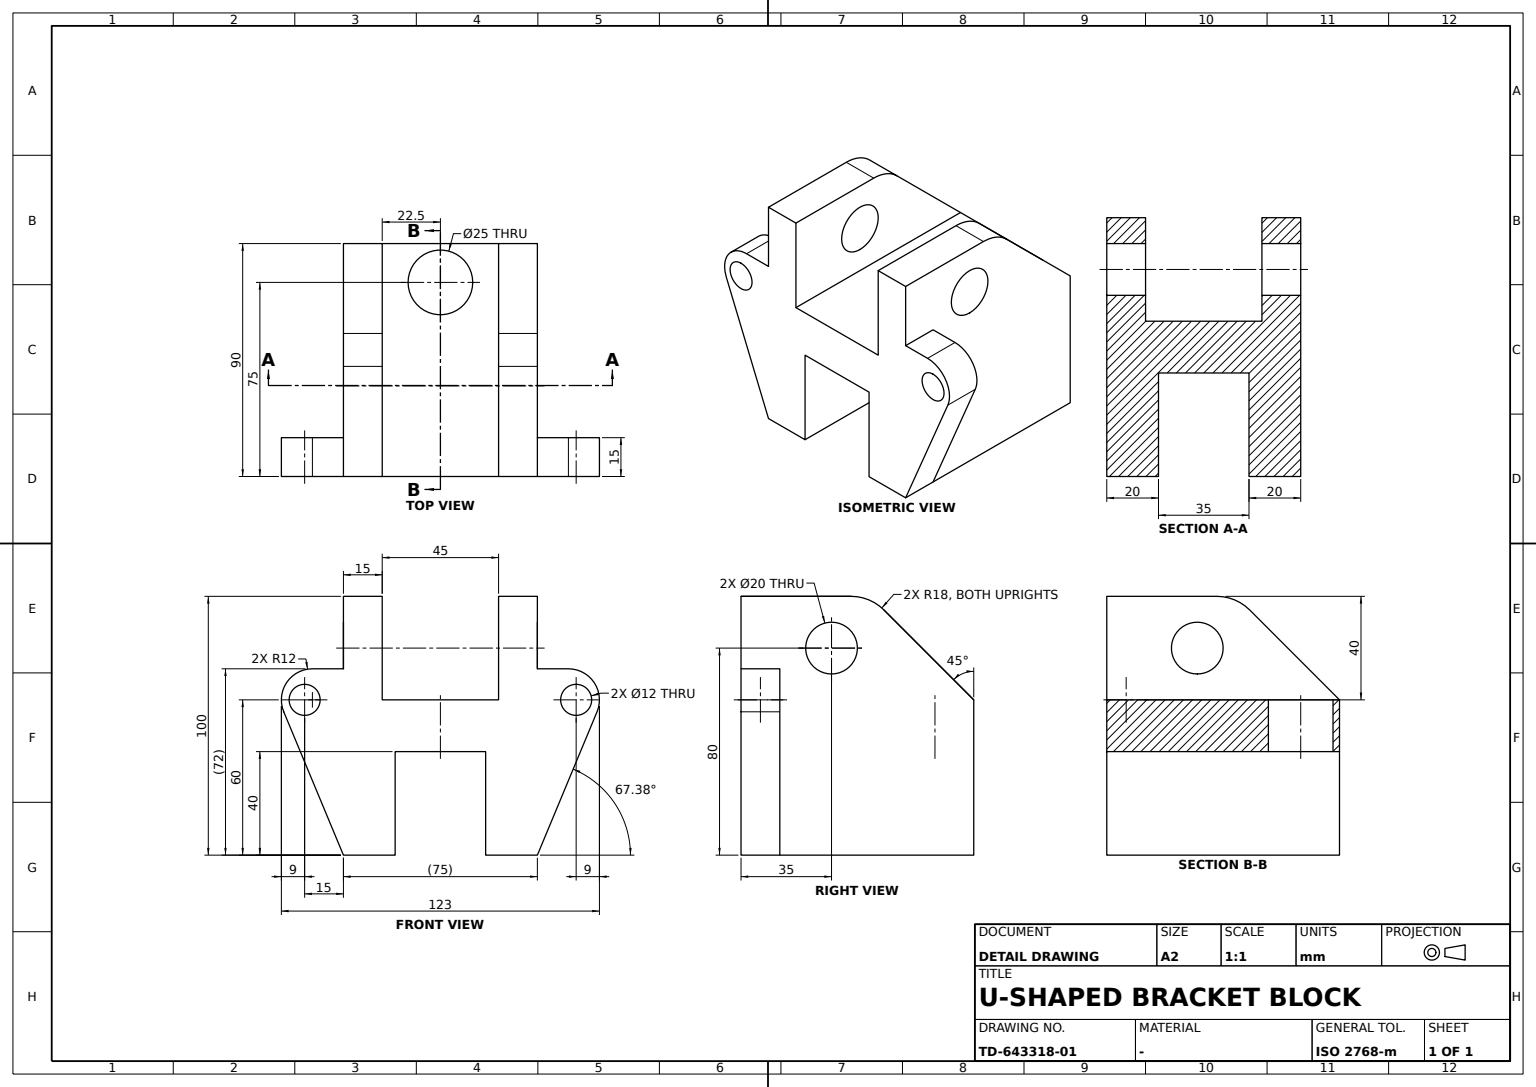
ISO-10303-21;
HEADER;
FILE_DESCRIPTION((''),'2;1');
FILE_NAME('','',(''),(''),'','','');
FILE_SCHEMA(('AUTOMOTIVE_DESIGN'));
ENDSEC;
DATA;
#1=APPLICATION_CONTEXT('');
#2=PRODUCT_CONTEXT('',#1,'mechanical');
#3=PRODUCT('','','',(#2));
#4=PRODUCT_DEFINITION_FORMATION('','',#3);
#5=PRODUCT_DEFINITION_CONTEXT('',#1,'design');
#6=PRODUCT_DEFINITION('','',#4,#5);
#7=PRODUCT_DEFINITION_SHAPE('','',#6);
#8=(LENGTH_UNIT()NAMED_UNIT(*)SI_UNIT(.MILLI.,.METRE.));
#9=(NAMED_UNIT(*)PLANE_ANGLE_UNIT()SI_UNIT($,.RADIAN.));
#10=(NAMED_UNIT(*)SI_UNIT($,.STERADIAN.)SOLID_ANGLE_UNIT());
#11=UNCERTAINTY_MEASURE_WITH_UNIT(LENGTH_MEASURE(0.005),#8,'distance_accuracy_value','');
#12=(GEOMETRIC_REPRESENTATION_CONTEXT(3)GLOBAL_UNCERTAINTY_ASSIGNED_CONTEXT((#11))GLOBAL_UNIT_ASSIGNED_CONTEXT((#8,#9,#10))REPRESENTATION_CONTEXT('',''));
#13=CARTESIAN_POINT('',(60.576923,-45.,15.384615));
#14=VERTEX_POINT('',#13);
#15=CARTESIAN_POINT('',(60.576923,-30.,15.384615));
#16=VERTEX_POINT('',#15);
#17=CARTESIAN_POINT('',(60.576923,-37.5,15.384615));
#18=DIRECTION('',(0.,1.,0.));
#19=VECTOR('',#18,1000.);
#20=LINE('',#17,#19);
#21=EDGE_CURVE('',#14,#16,#20,.T.);
#22=ORIENTED_EDGE('',*,*,#21,.F.);
#23=CARTESIAN_POINT('',(37.5,-45.,-40.));
#24=VERTEX_POINT('',#23);
#25=CARTESIAN_POINT('',(46.153846,-45.,-19.230769));
#26=DIRECTION('',(-0.384615385,0.,-0.923076923));
#27=VECTOR('',#26,1000.);
#28=LINE('',#25,#27);
#29=EDGE_CURVE('',#14,#24,#28,.T.);
#30=ORIENTED_EDGE('',*,*,#29,.T.);
#31=CARTESIAN_POINT('',(37.5,-30.,-40.));
#32=VERTEX_POINT('',#31);
#33=CARTESIAN_POINT('',(37.5,0.,-40.));
#34=LINE('',#33,#19);
#35=EDGE_CURVE('',#24,#32,#34,.T.);
#36=ORIENTED_EDGE('',*,*,#35,.T.);
#37=CARTESIAN_POINT('',(67.5,-30.,32.));
#38=LINE('',#37,#27);
#39=EDGE_CURVE('',#16,#32,#38,.T.);
#40=ORIENTED_EDGE('',*,*,#39,.F.);
#41=EDGE_LOOP('',(#22,#30,#36,#40));
#42=FACE_BOUND('',#41,.T.);
#43=CARTESIAN_POINT('',(67.5,-45.,32.));
#44=DIRECTION('',(0.923076923,0.,-0.384615385));
#45=AXIS2_PLACEMENT_3D('',#43,#44,#26);
#46=PLANE('',#45);
#47=ADVANCED_FACE('',(#42),#46,.T.);
#48=CARTESIAN_POINT('',(-22.5,-10.,30.));
#49=VERTEX_POINT('',#48);
#50=CARTESIAN_POINT('',(-22.5,-10.,40.));
#51=DIRECTION('',(1.,0.,0.));
#52=DIRECTION('',(0.,0.,-1.));
#53=AXIS2_PLACEMENT_3D('',#50,#51,#52);
#54=CIRCLE('',#53,10.);
#55=EDGE_CURVE('',#49,#49,#54,.T.);
#56=ORIENTED_EDGE('',*,*,#55,.T.);
#57=EDGE_LOOP('',(#56));
#58=FACE_BOUND('',#57,.T.);
#59=CARTESIAN_POINT('',(-37.5,-10.,30.));
#60=VERTEX_POINT('',#59);
#61=CARTESIAN_POINT('',(-37.5,-10.,40.));
#62=AXIS2_PLACEMENT_3D('',#61,#51,#52);
#63=CIRCLE('',#62,10.);
#64=EDGE_CURVE('',#60,#60,#63,.T.);
#65=ORIENTED_EDGE('',*,*,#64,.F.);
#66=EDGE_LOOP('',(#65));
#67=FACE_BOUND('',#66,.T.);
#68=CARTESIAN_POINT('',(30.,-10.,40.));
#69=AXIS2_PLACEMENT_3D('',#68,#51,#18);
#70=CYLINDRICAL_SURFACE('',#69,10.);
#71=ADVANCED_FACE('',(#58,#67),#70,.F.);
#72=CARTESIAN_POINT('',(-12.5,30.,20.));
#73=VERTEX_POINT('',#72);
#74=CARTESIAN_POINT('',(0.,30.,20.));
#75=DIRECTION('',(-1.,0.,0.));
#76=AXIS2_PLACEMENT_3D('',#74,#52,#75);
#77=CIRCLE('',#76,12.5);
#78=EDGE_CURVE('',#73,#73,#77,.F.);
#79=ORIENTED_EDGE('',*,*,#78,.T.);
#80=EDGE_LOOP('',(#79));
#81=FACE_BOUND('',#80,.T.);
#82=CARTESIAN_POINT('',(12.5,30.,0.));
#83=VERTEX_POINT('',#82);
#84=CARTESIAN_POINT('',(0.,30.,0.));
#85=DIRECTION('',(0.,0.,1.));
#86=AXIS2_PLACEMENT_3D('',#84,#85,#51);
#87=CIRCLE('',#86,12.5);
#88=EDGE_CURVE('',#83,#83,#87,.T.);
#89=ORIENTED_EDGE('',*,*,#88,.F.);
#90=EDGE_LOOP('',(#89));
#91=FACE_BOUND('',#90,.T.);
#92=CARTESIAN_POINT('',(0.,30.,10.));
#93=AXIS2_PLACEMENT_3D('',#92,#85,#18);
#94=CYLINDRICAL_SURFACE('',#93,12.5);
#95=ADVANCED_FACE('',(#81,#91),#94,.F.);
#96=CARTESIAN_POINT('',(37.5,-10.,50.));
#97=VERTEX_POINT('',#96);
#98=CARTESIAN_POINT('',(37.5,-10.,40.));
#99=AXIS2_PLACEMENT_3D('',#98,#75,#85);
#100=CIRCLE('',#99,10.);
#101=EDGE_CURVE('',#97,#97,#100,.F.);
#102=ORIENTED_EDGE('',*,*,#101,.T.);
#103=EDGE_LOOP('',(#102));
#104=FACE_BOUND('',#103,.T.);
#105=CARTESIAN_POINT('',(22.5,-10.,30.));
#106=VERTEX_POINT('',#105);
#107=CARTESIAN_POINT('',(22.5,-10.,40.));
#108=AXIS2_PLACEMENT_3D('',#107,#51,#52);
#109=CIRCLE('',#108,10.);
#110=EDGE_CURVE('',#106,#106,#109,.T.);
#111=ORIENTED_EDGE('',*,*,#110,.F.);
#112=EDGE_LOOP('',(#111));
#113=FACE_BOUND('',#112,.T.);
#114=ADVANCED_FACE('',(#104,#113),#70,.F.);
#115=CARTESIAN_POINT('',(-22.5,10.272078,54.727922));
#116=VERTEX_POINT('',#115);
#117=CARTESIAN_POINT('',(-37.5,10.272078,54.727922));
#118=VERTEX_POINT('',#117);
#119=CARTESIAN_POINT('',(-30.,10.272078,54.727922));
#120=VECTOR('',#75,1000.);
#121=LINE('',#119,#120);
#122=EDGE_CURVE('',#116,#118,#121,.T.);
#123=ORIENTED_EDGE('',*,*,#122,.T.);
#124=CARTESIAN_POINT('',(-37.5,-2.455844,60.));
#125=VERTEX_POINT('',#124);
#126=CARTESIAN_POINT('',(-37.5,-2.455844,42.));
#127=AXIS2_PLACEMENT_3D('',#126,#51,#52);
#128=CIRCLE('',#127,18.);
#129=EDGE_CURVE('',#118,#125,#128,.T.);
#130=ORIENTED_EDGE('',*,*,#129,.T.);
#131=CARTESIAN_POINT('',(-22.5,-2.455844,60.));
#132=VERTEX_POINT('',#131);
#133=CARTESIAN_POINT('',(-30.,-2.455844,60.));
#134=LINE('',#133,#120);
#135=EDGE_CURVE('',#132,#125,#134,.T.);
#136=ORIENTED_EDGE('',*,*,#135,.F.);
#137=CARTESIAN_POINT('',(-22.5,-2.455844,42.));
#138=AXIS2_PLACEMENT_3D('',#137,#51,#52);
#139=CIRCLE('',#138,18.);
#140=EDGE_CURVE('',#116,#132,#139,.T.);
#141=ORIENTED_EDGE('',*,*,#140,.F.);
#142=EDGE_LOOP('',(#123,#130,#136,#141));
#143=FACE_BOUND('',#142,.T.);
#144=CARTESIAN_POINT('',(-30.,-2.455844,42.));
#145=AXIS2_PLACEMENT_3D('',#144,#75,#85);
#146=CYLINDRICAL_SURFACE('',#145,18.);
#147=ADVANCED_FACE('',(#143),#146,.T.);
#148=ORIENTED_EDGE('',*,*,#122,.F.);
#149=CARTESIAN_POINT('',(-22.5,45.,20.));
#150=VERTEX_POINT('',#149);
#151=CARTESIAN_POINT('',(-22.5,5.,60.));
#152=DIRECTION('',(0.,0.707106781,-0.707106781));
#153=VECTOR('',#152,1000.);
#154=LINE('',#151,#153);
#155=EDGE_CURVE('',#116,#150,#154,.T.);
#156=ORIENTED_EDGE('',*,*,#155,.T.);
#157=CARTESIAN_POINT('',(-37.5,45.,20.));
#158=VERTEX_POINT('',#157);
#159=CARTESIAN_POINT('',(0.,45.,20.));
#160=VECTOR('',#51,1000.);
#161=LINE('',#159,#160);
#162=EDGE_CURVE('',#158,#150,#161,.T.);
#163=ORIENTED_EDGE('',*,*,#162,.F.);
#164=CARTESIAN_POINT('',(-37.5,5.,60.));
#165=LINE('',#164,#153);
#166=EDGE_CURVE('',#118,#158,#165,.T.);
#167=ORIENTED_EDGE('',*,*,#166,.F.);
#168=EDGE_LOOP('',(#148,#156,#163,#167));
#169=FACE_BOUND('',#168,.T.);
#170=CARTESIAN_POINT('',(37.5,5.,60.));
#171=DIRECTION('',(0.,0.707106781,0.707106781));
#172=AXIS2_PLACEMENT_3D('',#170,#171,#152);
#173=PLANE('',#172);
#174=ADVANCED_FACE('',(#169),#173,.T.);
#175=CARTESIAN_POINT('',(17.5,45.,0.));
#176=VERTEX_POINT('',#175);
#177=CARTESIAN_POINT('',(17.5,45.,-40.));
#178=VERTEX_POINT('',#177);
#179=VECTOR('',#52,1000.);
#180=LINE('',#175,#179);
#181=EDGE_CURVE('',#176,#178,#180,.T.);
#182=ORIENTED_EDGE('',*,*,#181,.F.);
#183=CARTESIAN_POINT('',(-17.5,45.,0.));
#184=VERTEX_POINT('',#183);
#185=CARTESIAN_POINT('',(0.,45.,0.));
#186=LINE('',#185,#160);
#187=EDGE_CURVE('',#184,#176,#186,.T.);
#188=ORIENTED_EDGE('',*,*,#187,.F.);
#189=CARTESIAN_POINT('',(-17.5,45.,-40.));
#190=VERTEX_POINT('',#189);
#191=VECTOR('',#85,1000.);
#192=LINE('',#183,#191);
#193=EDGE_CURVE('',#190,#184,#192,.T.);
#194=ORIENTED_EDGE('',*,*,#193,.F.);
#195=CARTESIAN_POINT('',(-37.5,45.,-40.));
#196=VERTEX_POINT('',#195);
#197=CARTESIAN_POINT('',(0.,45.,-40.));
#198=LINE('',#197,#160);
#199=EDGE_CURVE('',#196,#190,#198,.T.);
#200=ORIENTED_EDGE('',*,*,#199,.F.);
#201=CARTESIAN_POINT('',(-37.5,45.,0.));
#202=LINE('',#201,#179);
#203=EDGE_CURVE('',#158,#196,#202,.T.);
#204=ORIENTED_EDGE('',*,*,#203,.F.);
#205=ORIENTED_EDGE('',*,*,#162,.T.);
#206=CARTESIAN_POINT('',(22.5,45.,20.));
#207=VERTEX_POINT('',#206);
#208=LINE('',#159,#120);
#209=EDGE_CURVE('',#207,#150,#208,.T.);
#210=ORIENTED_EDGE('',*,*,#209,.F.);
#211=CARTESIAN_POINT('',(37.5,45.,20.));
#212=VERTEX_POINT('',#211);
#213=LINE('',#211,#120);
#214=EDGE_CURVE('',#212,#207,#213,.T.);
#215=ORIENTED_EDGE('',*,*,#214,.F.);
#216=CARTESIAN_POINT('',(37.5,45.,-40.));
#217=VERTEX_POINT('',#216);
#218=CARTESIAN_POINT('',(37.5,45.,0.));
#219=LINE('',#218,#191);
#220=EDGE_CURVE('',#217,#212,#219,.T.);
#221=ORIENTED_EDGE('',*,*,#220,.F.);
#222=EDGE_CURVE('',#178,#217,#198,.T.);
#223=ORIENTED_EDGE('',*,*,#222,.F.);
#224=EDGE_LOOP('',(#182,#188,#194,#200,#204,#205,#210,#215,#221,#223));
#225=FACE_BOUND('',#224,.T.);
#226=AXIS2_PLACEMENT_3D('',#185,#18,#75);
#227=PLANE('',#226);
#228=ADVANCED_FACE('',(#225),#227,.T.);
#229=CARTESIAN_POINT('',(-37.5,-45.,-40.));
#230=VERTEX_POINT('',#229);
#231=CARTESIAN_POINT('',(-17.5,-45.,-40.));
#232=VERTEX_POINT('',#231);
#233=CARTESIAN_POINT('',(0.,-45.,-40.));
#234=LINE('',#233,#160);
#235=EDGE_CURVE('',#230,#232,#234,.T.);
#236=ORIENTED_EDGE('',*,*,#235,.F.);
#237=CARTESIAN_POINT('',(-37.5,-30.,-40.));
#238=VERTEX_POINT('',#237);
#239=CARTESIAN_POINT('',(-37.5,0.,-40.));
#240=LINE('',#239,#19);
#241=EDGE_CURVE('',#230,#238,#240,.T.);
#242=ORIENTED_EDGE('',*,*,#241,.T.);
#243=EDGE_CURVE('',#238,#196,#240,.T.);
#244=ORIENTED_EDGE('',*,*,#243,.T.);
#245=ORIENTED_EDGE('',*,*,#199,.T.);
#246=CARTESIAN_POINT('',(-17.5,0.,-40.));
#247=LINE('',#246,#19);
#248=EDGE_CURVE('',#232,#190,#247,.T.);
#249=ORIENTED_EDGE('',*,*,#248,.F.);
#250=EDGE_LOOP('',(#236,#242,#244,#245,#249));
#251=FACE_BOUND('',#250,.T.);
#252=AXIS2_PLACEMENT_3D('',#239,#85,#51);
#253=PLANE('',#252);
#254=ADVANCED_FACE('',(#251),#253,.F.);
#255=CARTESIAN_POINT('',(-37.5,-45.,60.));
#256=VERTEX_POINT('',#255);
#257=CARTESIAN_POINT('',(-22.5,-45.,60.));
#258=VERTEX_POINT('',#257);
#259=CARTESIAN_POINT('',(0.,-45.,60.));
#260=LINE('',#259,#160);
#261=EDGE_CURVE('',#256,#258,#260,.T.);
#262=ORIENTED_EDGE('',*,*,#261,.T.);
#263=LINE('',#257,#19);
#264=EDGE_CURVE('',#258,#132,#263,.T.);
#265=ORIENTED_EDGE('',*,*,#264,.T.);
#266=ORIENTED_EDGE('',*,*,#135,.T.);
#267=LINE('',#255,#19);
#268=EDGE_CURVE('',#256,#125,#267,.T.);
#269=ORIENTED_EDGE('',*,*,#268,.F.);
#270=EDGE_LOOP('',(#262,#265,#266,#269));
#271=FACE_BOUND('',#270,.T.);
#272=CARTESIAN_POINT('',(37.5,-45.,60.));
#273=AXIS2_PLACEMENT_3D('',#272,#85,#18);
#274=PLANE('',#273);
#275=ADVANCED_FACE('',(#271),#274,.T.);
#276=ORIENTED_EDGE('',*,*,#264,.F.);
#277=CARTESIAN_POINT('',(-22.5,-45.,20.));
#278=VERTEX_POINT('',#277);
#279=CARTESIAN_POINT('',(-22.5,-45.,0.));
#280=LINE('',#279,#191);
#281=EDGE_CURVE('',#278,#258,#280,.T.);
#282=ORIENTED_EDGE('',*,*,#281,.F.);
#283=CARTESIAN_POINT('',(-22.5,0.,20.));
#284=DIRECTION('',(0.,-1.,0.));
#285=VECTOR('',#284,1000.);
#286=LINE('',#283,#285);
#287=EDGE_CURVE('',#150,#278,#286,.T.);
#288=ORIENTED_EDGE('',*,*,#287,.F.);
#289=ORIENTED_EDGE('',*,*,#155,.F.);
#290=ORIENTED_EDGE('',*,*,#140,.T.);
#291=EDGE_LOOP('',(#276,#282,#288,#289,#290));
#292=FACE_BOUND('',#291,.T.);
#293=ORIENTED_EDGE('',*,*,#55,.F.);
#294=EDGE_LOOP('',(#293));
#295=FACE_BOUND('',#294,.T.);
#296=CARTESIAN_POINT('',(-22.5,0.,0.));
#297=AXIS2_PLACEMENT_3D('',#296,#51,#18);
#298=PLANE('',#297);
#299=ADVANCED_FACE('',(#292,#295),#298,.T.);
#300=VERTEX_POINT('',#272);
#301=CARTESIAN_POINT('',(37.5,-2.455844,60.));
#302=VERTEX_POINT('',#301);
#303=CARTESIAN_POINT('',(37.5,0.,60.));
#304=LINE('',#303,#19);
#305=EDGE_CURVE('',#300,#302,#304,.T.);
#306=ORIENTED_EDGE('',*,*,#305,.F.);
#307=CARTESIAN_POINT('',(37.5,-45.,32.));
#308=VERTEX_POINT('',#307);
#309=CARTESIAN_POINT('',(37.5,-45.,0.));
#310=LINE('',#309,#191);
#311=EDGE_CURVE('',#308,#300,#310,.T.);
#312=ORIENTED_EDGE('',*,*,#311,.F.);
#313=CARTESIAN_POINT('',(37.5,-30.,32.));
#314=VERTEX_POINT('',#313);
#315=CARTESIAN_POINT('',(37.5,0.,32.));
#316=LINE('',#315,#19);
#317=EDGE_CURVE('',#308,#314,#316,.T.);
#318=ORIENTED_EDGE('',*,*,#317,.T.);
#319=LINE('',#31,#191);
#320=EDGE_CURVE('',#32,#314,#319,.T.);
#321=ORIENTED_EDGE('',*,*,#320,.F.);
#322=EDGE_CURVE('',#32,#217,#34,.T.);
#323=ORIENTED_EDGE('',*,*,#322,.T.);
#324=ORIENTED_EDGE('',*,*,#220,.T.);
#325=CARTESIAN_POINT('',(37.5,10.272078,54.727922));
#326=VERTEX_POINT('',#325);
#327=CARTESIAN_POINT('',(37.5,52.5,12.5));
#328=LINE('',#327,#153);
#329=EDGE_CURVE('',#326,#212,#328,.T.);
#330=ORIENTED_EDGE('',*,*,#329,.F.);
#331=CARTESIAN_POINT('',(37.5,-2.455844,42.));
#332=AXIS2_PLACEMENT_3D('',#331,#75,#85);
#333=CIRCLE('',#332,18.);
#334=EDGE_CURVE('',#302,#326,#333,.T.);
#335=ORIENTED_EDGE('',*,*,#334,.F.);
#336=EDGE_LOOP('',(#306,#312,#318,#321,#323,#324,#330,#335));
#337=FACE_BOUND('',#336,.T.);
#338=ORIENTED_EDGE('',*,*,#101,.F.);
#339=EDGE_LOOP('',(#338));
#340=FACE_BOUND('',#339,.T.);
#341=AXIS2_PLACEMENT_3D('',#33,#75,#85);
#342=PLANE('',#341);
#343=ADVANCED_FACE('',(#337,#340),#342,.F.);
#344=CARTESIAN_POINT('',(-37.5,-45.,32.));
#345=VERTEX_POINT('',#344);
#346=CARTESIAN_POINT('',(-37.5,-30.,32.));
#347=VERTEX_POINT('',#346);
#348=LINE('',#344,#19);
#349=EDGE_CURVE('',#345,#347,#348,.T.);
#350=ORIENTED_EDGE('',*,*,#349,.F.);
#351=CARTESIAN_POINT('',(-37.5,-45.,0.));
#352=LINE('',#351,#179);
#353=EDGE_CURVE('',#256,#345,#352,.T.);
#354=ORIENTED_EDGE('',*,*,#353,.F.);
#355=ORIENTED_EDGE('',*,*,#268,.T.);
#356=ORIENTED_EDGE('',*,*,#129,.F.);
#357=ORIENTED_EDGE('',*,*,#166,.T.);
#358=ORIENTED_EDGE('',*,*,#203,.T.);
#359=ORIENTED_EDGE('',*,*,#243,.F.);
#360=CARTESIAN_POINT('',(-37.5,-30.,0.));
#361=LINE('',#360,#191);
#362=EDGE_CURVE('',#238,#347,#361,.T.);
#363=ORIENTED_EDGE('',*,*,#362,.T.);
#364=EDGE_LOOP('',(#350,#354,#355,#356,#357,#358,#359,#363));
#365=FACE_BOUND('',#364,.T.);
#366=ORIENTED_EDGE('',*,*,#64,.T.);
#367=EDGE_LOOP('',(#366));
#368=FACE_BOUND('',#367,.T.);
#369=CARTESIAN_POINT('',(-37.5,0.,20.));
#370=AXIS2_PLACEMENT_3D('',#369,#51,#52);
#371=PLANE('',#370);
#372=ADVANCED_FACE('',(#365,#368),#371,.F.);
#373=CARTESIAN_POINT('',(22.5,10.272078,54.727922));
#374=VERTEX_POINT('',#373);
#375=CARTESIAN_POINT('',(22.5,5.,60.));
#376=LINE('',#375,#153);
#377=EDGE_CURVE('',#374,#207,#376,.T.);
#378=ORIENTED_EDGE('',*,*,#377,.F.);
#379=EDGE_CURVE('',#326,#374,#121,.T.);
#380=ORIENTED_EDGE('',*,*,#379,.F.);
#381=ORIENTED_EDGE('',*,*,#329,.T.);
#382=ORIENTED_EDGE('',*,*,#214,.T.);
#383=EDGE_LOOP('',(#378,#380,#381,#382));
#384=FACE_BOUND('',#383,.T.);
#385=ADVANCED_FACE('',(#384),#173,.T.);
#386=CARTESIAN_POINT('',(17.5,-45.,0.));
#387=VERTEX_POINT('',#386);
#388=CARTESIAN_POINT('',(17.5,-45.,-40.));
#389=VERTEX_POINT('',#388);
#390=LINE('',#386,#179);
#391=EDGE_CURVE('',#387,#389,#390,.T.);
#392=ORIENTED_EDGE('',*,*,#391,.F.);
#393=CARTESIAN_POINT('',(17.5,0.,0.));
#394=LINE('',#393,#19);
#395=EDGE_CURVE('',#387,#176,#394,.T.);
#396=ORIENTED_EDGE('',*,*,#395,.T.);
#397=ORIENTED_EDGE('',*,*,#181,.T.);
#398=CARTESIAN_POINT('',(17.5,0.,-40.));
#399=LINE('',#398,#19);
#400=EDGE_CURVE('',#389,#178,#399,.T.);
#401=ORIENTED_EDGE('',*,*,#400,.F.);
#402=EDGE_LOOP('',(#392,#396,#397,#401));
#403=FACE_BOUND('',#402,.T.);
#404=AXIS2_PLACEMENT_3D('',#393,#51,#52);
#405=PLANE('',#404);
#406=ADVANCED_FACE('',(#403),#405,.F.);
#407=ORIENTED_EDGE('',*,*,#349,.T.);
#408=CARTESIAN_POINT('',(-49.5,-30.,32.));
#409=VERTEX_POINT('',#408);
#410=CARTESIAN_POINT('',(0.,-30.,32.));
#411=LINE('',#410,#120);
#412=EDGE_CURVE('',#347,#409,#411,.T.);
#413=ORIENTED_EDGE('',*,*,#412,.T.);
#414=CARTESIAN_POINT('',(-49.5,-45.,32.));
#415=VERTEX_POINT('',#414);
#416=CARTESIAN_POINT('',(-49.5,-37.5,32.));
#417=LINE('',#416,#19);
#418=EDGE_CURVE('',#415,#409,#417,.T.);
#419=ORIENTED_EDGE('',*,*,#418,.F.);
#420=LINE('',#307,#120);
#421=EDGE_CURVE('',#345,#415,#420,.T.);
#422=ORIENTED_EDGE('',*,*,#421,.F.);
#423=EDGE_LOOP('',(#407,#413,#419,#422));
#424=FACE_BOUND('',#423,.T.);
#425=AXIS2_PLACEMENT_3D('',#307,#85,#51);
#426=PLANE('',#425);
#427=ADVANCED_FACE('',(#424),#426,.T.);
#428=ORIENTED_EDGE('',*,*,#261,.F.);
#429=ORIENTED_EDGE('',*,*,#353,.T.);
#430=ORIENTED_EDGE('',*,*,#421,.T.);
#431=CARTESIAN_POINT('',(-60.576923,-45.,15.384615));
#432=VERTEX_POINT('',#431);
#433=CARTESIAN_POINT('',(-49.5,-45.,20.));
#434=AXIS2_PLACEMENT_3D('',#433,#18,#85);
#435=CIRCLE('',#434,12.);
#436=EDGE_CURVE('',#432,#415,#435,.T.);
#437=ORIENTED_EDGE('',*,*,#436,.F.);
#438=CARTESIAN_POINT('',(-46.153846,-45.,-19.230769));
#439=DIRECTION('',(0.384615385,0.,-0.923076923));
#440=VECTOR('',#439,1000.);
#441=LINE('',#438,#440);
#442=EDGE_CURVE('',#432,#230,#441,.T.);
#443=ORIENTED_EDGE('',*,*,#442,.T.);
#444=ORIENTED_EDGE('',*,*,#235,.T.);
#445=CARTESIAN_POINT('',(-17.5,-45.,0.));
#446=VERTEX_POINT('',#445);
#447=LINE('',#445,#191);
#448=EDGE_CURVE('',#232,#446,#447,.T.);
#449=ORIENTED_EDGE('',*,*,#448,.T.);
#450=CARTESIAN_POINT('',(0.,-45.,0.));
#451=LINE('',#450,#160);
#452=EDGE_CURVE('',#446,#387,#451,.T.);
#453=ORIENTED_EDGE('',*,*,#452,.T.);
#454=ORIENTED_EDGE('',*,*,#391,.T.);
#455=EDGE_CURVE('',#389,#24,#234,.T.);
#456=ORIENTED_EDGE('',*,*,#455,.T.);
#457=ORIENTED_EDGE('',*,*,#29,.F.);
#458=CARTESIAN_POINT('',(49.5,-45.,32.));
#459=VERTEX_POINT('',#458);
#460=CARTESIAN_POINT('',(49.5,-45.,20.));
#461=AXIS2_PLACEMENT_3D('',#460,#18,#85);
#462=CIRCLE('',#461,12.);
#463=EDGE_CURVE('',#459,#14,#462,.T.);
#464=ORIENTED_EDGE('',*,*,#463,.F.);
#465=CARTESIAN_POINT('',(0.,-45.,32.));
#466=LINE('',#465,#160);
#467=EDGE_CURVE('',#308,#459,#466,.T.);
#468=ORIENTED_EDGE('',*,*,#467,.F.);
#469=ORIENTED_EDGE('',*,*,#311,.T.);
#470=CARTESIAN_POINT('',(22.5,-45.,60.));
#471=VERTEX_POINT('',#470);
#472=LINE('',#272,#120);
#473=EDGE_CURVE('',#300,#471,#472,.T.);
#474=ORIENTED_EDGE('',*,*,#473,.T.);
#475=CARTESIAN_POINT('',(22.5,-45.,20.));
#476=VERTEX_POINT('',#475);
#477=CARTESIAN_POINT('',(22.5,-45.,0.));
#478=LINE('',#477,#191);
#479=EDGE_CURVE('',#476,#471,#478,.T.);
#480=ORIENTED_EDGE('',*,*,#479,.F.);
#481=CARTESIAN_POINT('',(0.,-45.,20.));
#482=LINE('',#481,#120);
#483=EDGE_CURVE('',#476,#278,#482,.T.);
#484=ORIENTED_EDGE('',*,*,#483,.T.);
#485=ORIENTED_EDGE('',*,*,#281,.T.);
#486=EDGE_LOOP('',(#428,#429,#430,#437,#443,#444,#449,#453,#454,#456,#457,#464,#468,#469,#474,#480,#484,#485));
#487=FACE_BOUND('',#486,.T.);
#488=CARTESIAN_POINT('',(-52.5,-45.,26.));
#489=VERTEX_POINT('',#488);
#490=CARTESIAN_POINT('',(-52.5,-45.,20.));
#491=AXIS2_PLACEMENT_3D('',#490,#18,#85);
#492=CIRCLE('',#491,6.);
#493=EDGE_CURVE('',#489,#489,#492,.T.);
#494=ORIENTED_EDGE('',*,*,#493,.T.);
#495=EDGE_LOOP('',(#494));
#496=FACE_BOUND('',#495,.T.);
#497=CARTESIAN_POINT('',(52.5,-45.,26.));
#498=VERTEX_POINT('',#497);
#499=CARTESIAN_POINT('',(52.5,-45.,20.));
#500=AXIS2_PLACEMENT_3D('',#499,#18,#85);
#501=CIRCLE('',#500,6.);
#502=EDGE_CURVE('',#498,#498,#501,.F.);
#503=ORIENTED_EDGE('',*,*,#502,.F.);
#504=EDGE_LOOP('',(#503));
#505=FACE_BOUND('',#504,.T.);
#506=AXIS2_PLACEMENT_3D('',#450,#18,#75);
#507=PLANE('',#506);
#508=ADVANCED_FACE('',(#487,#496,#505),#507,.F.);
#509=ORIENTED_EDGE('',*,*,#110,.T.);
#510=EDGE_LOOP('',(#509));
#511=FACE_BOUND('',#510,.T.);
#512=CARTESIAN_POINT('',(22.5,-2.455844,60.));
#513=VERTEX_POINT('',#512);
#514=LINE('',#470,#19);
#515=EDGE_CURVE('',#471,#513,#514,.T.);
#516=ORIENTED_EDGE('',*,*,#515,.T.);
#517=CARTESIAN_POINT('',(22.5,-2.455844,42.));
#518=AXIS2_PLACEMENT_3D('',#517,#51,#52);
#519=CIRCLE('',#518,18.);
#520=EDGE_CURVE('',#374,#513,#519,.T.);
#521=ORIENTED_EDGE('',*,*,#520,.F.);
#522=ORIENTED_EDGE('',*,*,#377,.T.);
#523=CARTESIAN_POINT('',(22.5,0.,20.));
#524=LINE('',#523,#285);
#525=EDGE_CURVE('',#207,#476,#524,.T.);
#526=ORIENTED_EDGE('',*,*,#525,.T.);
#527=ORIENTED_EDGE('',*,*,#479,.T.);
#528=EDGE_LOOP('',(#516,#521,#522,#526,#527));
#529=FACE_BOUND('',#528,.T.);
#530=CARTESIAN_POINT('',(22.5,0.,0.));
#531=AXIS2_PLACEMENT_3D('',#530,#51,#18);
#532=PLANE('',#531);
#533=ADVANCED_FACE('',(#511,#529),#532,.F.);
#534=CARTESIAN_POINT('',(-60.576923,-30.,15.384615));
#535=VERTEX_POINT('',#534);
#536=CARTESIAN_POINT('',(-67.5,-30.,32.));
#537=LINE('',#536,#440);
#538=EDGE_CURVE('',#535,#238,#537,.T.);
#539=ORIENTED_EDGE('',*,*,#538,.T.);
#540=ORIENTED_EDGE('',*,*,#241,.F.);
#541=ORIENTED_EDGE('',*,*,#442,.F.);
#542=CARTESIAN_POINT('',(-60.576923,-37.5,15.384615));
#543=LINE('',#542,#19);
#544=EDGE_CURVE('',#432,#535,#543,.T.);
#545=ORIENTED_EDGE('',*,*,#544,.T.);
#546=EDGE_LOOP('',(#539,#540,#541,#545));
#547=FACE_BOUND('',#546,.T.);
#548=CARTESIAN_POINT('',(-67.5,-45.,32.));
#549=DIRECTION('',(0.923076923,0.,0.384615385));
#550=AXIS2_PLACEMENT_3D('',#548,#549,#439);
#551=PLANE('',#550);
#552=ADVANCED_FACE('',(#547),#551,.F.);
#553=CARTESIAN_POINT('',(-17.5,0.,0.));
#554=LINE('',#553,#19);
#555=EDGE_CURVE('',#446,#184,#554,.T.);
#556=ORIENTED_EDGE('',*,*,#555,.F.);
#557=ORIENTED_EDGE('',*,*,#448,.F.);
#558=ORIENTED_EDGE('',*,*,#248,.T.);
#559=ORIENTED_EDGE('',*,*,#193,.T.);
#560=EDGE_LOOP('',(#556,#557,#558,#559));
#561=FACE_BOUND('',#560,.T.);
#562=AXIS2_PLACEMENT_3D('',#246,#75,#85);
#563=PLANE('',#562);
#564=ADVANCED_FACE('',(#561),#563,.F.);
#565=ORIENTED_EDGE('',*,*,#520,.T.);
#566=EDGE_CURVE('',#302,#513,#134,.T.);
#567=ORIENTED_EDGE('',*,*,#566,.F.);
#568=ORIENTED_EDGE('',*,*,#334,.T.);
#569=ORIENTED_EDGE('',*,*,#379,.T.);
#570=EDGE_LOOP('',(#565,#567,#568,#569));
#571=FACE_BOUND('',#570,.T.);
#572=ADVANCED_FACE('',(#571),#146,.T.);
#573=ORIENTED_EDGE('',*,*,#287,.T.);
#574=ORIENTED_EDGE('',*,*,#483,.F.);
#575=ORIENTED_EDGE('',*,*,#525,.F.);
#576=ORIENTED_EDGE('',*,*,#209,.T.);
#577=EDGE_LOOP('',(#573,#574,#575,#576));
#578=FACE_BOUND('',#577,.T.);
#579=ORIENTED_EDGE('',*,*,#78,.F.);
#580=EDGE_LOOP('',(#579));
#581=FACE_BOUND('',#580,.T.);
#582=CARTESIAN_POINT('',(37.5,0.,20.));
#583=AXIS2_PLACEMENT_3D('',#582,#52,#75);
#584=PLANE('',#583);
#585=ADVANCED_FACE('',(#578,#581),#584,.F.);
#586=ORIENTED_EDGE('',*,*,#322,.F.);
#587=ORIENTED_EDGE('',*,*,#35,.F.);
#588=ORIENTED_EDGE('',*,*,#455,.F.);
#589=ORIENTED_EDGE('',*,*,#400,.T.);
#590=ORIENTED_EDGE('',*,*,#222,.T.);
#591=EDGE_LOOP('',(#586,#587,#588,#589,#590));
#592=FACE_BOUND('',#591,.T.);
#593=ADVANCED_FACE('',(#592),#253,.F.);
#594=ORIENTED_EDGE('',*,*,#39,.T.);
#595=ORIENTED_EDGE('',*,*,#320,.T.);
#596=CARTESIAN_POINT('',(49.5,-30.,32.));
#597=VERTEX_POINT('',#596);
#598=LINE('',#313,#160);
#599=EDGE_CURVE('',#314,#597,#598,.T.);
#600=ORIENTED_EDGE('',*,*,#599,.T.);
#601=CARTESIAN_POINT('',(49.5,-30.,20.));
#602=AXIS2_PLACEMENT_3D('',#601,#284,#52);
#603=CIRCLE('',#602,12.);
#604=EDGE_CURVE('',#16,#597,#603,.T.);
#605=ORIENTED_EDGE('',*,*,#604,.F.);
#606=EDGE_LOOP('',(#594,#595,#600,#605));
#607=FACE_BOUND('',#606,.T.);
#608=CARTESIAN_POINT('',(52.5,-30.,14.));
#609=VERTEX_POINT('',#608);
#610=CARTESIAN_POINT('',(52.5,-30.,20.));
#611=AXIS2_PLACEMENT_3D('',#610,#284,#52);
#612=CIRCLE('',#611,6.);
#613=EDGE_CURVE('',#609,#609,#612,.T.);
#614=ORIENTED_EDGE('',*,*,#613,.T.);
#615=EDGE_LOOP('',(#614));
#616=FACE_BOUND('',#615,.T.);
#617=CARTESIAN_POINT('',(0.,-30.,0.));
#618=AXIS2_PLACEMENT_3D('',#617,#284,#51);
#619=PLANE('',#618);
#620=ADVANCED_FACE('',(#607,#616),#619,.F.);
#621=ORIENTED_EDGE('',*,*,#599,.F.);
#622=ORIENTED_EDGE('',*,*,#317,.F.);
#623=ORIENTED_EDGE('',*,*,#467,.T.);
#624=CARTESIAN_POINT('',(49.5,-37.5,32.));
#625=LINE('',#624,#19);
#626=EDGE_CURVE('',#459,#597,#625,.T.);
#627=ORIENTED_EDGE('',*,*,#626,.T.);
#628=EDGE_LOOP('',(#621,#622,#623,#627));
#629=FACE_BOUND('',#628,.T.);
#630=ADVANCED_FACE('',(#629),#426,.T.);
#631=ORIENTED_EDGE('',*,*,#412,.F.);
#632=ORIENTED_EDGE('',*,*,#362,.F.);
#633=ORIENTED_EDGE('',*,*,#538,.F.);
#634=CARTESIAN_POINT('',(-49.5,-30.,20.));
#635=AXIS2_PLACEMENT_3D('',#634,#284,#52);
#636=CIRCLE('',#635,12.);
#637=EDGE_CURVE('',#409,#535,#636,.T.);
#638=ORIENTED_EDGE('',*,*,#637,.F.);
#639=EDGE_LOOP('',(#631,#632,#633,#638));
#640=FACE_BOUND('',#639,.T.);
#641=CARTESIAN_POINT('',(-52.5,-30.,14.));
#642=VERTEX_POINT('',#641);
#643=CARTESIAN_POINT('',(-52.5,-30.,20.));
#644=AXIS2_PLACEMENT_3D('',#643,#284,#52);
#645=CIRCLE('',#644,6.);
#646=EDGE_CURVE('',#642,#642,#645,.F.);
#647=ORIENTED_EDGE('',*,*,#646,.F.);
#648=EDGE_LOOP('',(#647));
#649=FACE_BOUND('',#648,.T.);
#650=ADVANCED_FACE('',(#640,#649),#619,.F.);
#651=ORIENTED_EDGE('',*,*,#88,.T.);
#652=EDGE_LOOP('',(#651));
#653=FACE_BOUND('',#652,.T.);
#654=ORIENTED_EDGE('',*,*,#452,.F.);
#655=ORIENTED_EDGE('',*,*,#555,.T.);
#656=ORIENTED_EDGE('',*,*,#187,.T.);
#657=ORIENTED_EDGE('',*,*,#395,.F.);
#658=EDGE_LOOP('',(#654,#655,#656,#657));
#659=FACE_BOUND('',#658,.T.);
#660=AXIS2_PLACEMENT_3D('',#553,#85,#51);
#661=PLANE('',#660);
#662=ADVANCED_FACE('',(#653,#659),#661,.F.);
#663=ORIENTED_EDGE('',*,*,#436,.T.);
#664=ORIENTED_EDGE('',*,*,#418,.T.);
#665=ORIENTED_EDGE('',*,*,#637,.T.);
#666=ORIENTED_EDGE('',*,*,#544,.F.);
#667=EDGE_LOOP('',(#663,#664,#665,#666));
#668=FACE_BOUND('',#667,.T.);
#669=CARTESIAN_POINT('',(-49.5,-37.5,20.));
#670=AXIS2_PLACEMENT_3D('',#669,#18,#85);
#671=CYLINDRICAL_SURFACE('',#670,12.);
#672=ADVANCED_FACE('',(#668),#671,.T.);
#673=ORIENTED_EDGE('',*,*,#502,.T.);
#674=EDGE_LOOP('',(#673));
#675=FACE_BOUND('',#674,.T.);
#676=ORIENTED_EDGE('',*,*,#613,.F.);
#677=EDGE_LOOP('',(#676));
#678=FACE_BOUND('',#677,.T.);
#679=CARTESIAN_POINT('',(52.5,-37.5,20.));
#680=AXIS2_PLACEMENT_3D('',#679,#284,#51);
#681=CYLINDRICAL_SURFACE('',#680,6.);
#682=ADVANCED_FACE('',(#675,#678),#681,.F.);
#683=ORIENTED_EDGE('',*,*,#463,.T.);
#684=ORIENTED_EDGE('',*,*,#21,.T.);
#685=ORIENTED_EDGE('',*,*,#604,.T.);
#686=ORIENTED_EDGE('',*,*,#626,.F.);
#687=EDGE_LOOP('',(#683,#684,#685,#686));
#688=FACE_BOUND('',#687,.T.);
#689=CARTESIAN_POINT('',(49.5,-37.5,20.));
#690=AXIS2_PLACEMENT_3D('',#689,#18,#44);
#691=CYLINDRICAL_SURFACE('',#690,12.);
#692=ADVANCED_FACE('',(#688),#691,.T.);
#693=ORIENTED_EDGE('',*,*,#473,.F.);
#694=ORIENTED_EDGE('',*,*,#305,.T.);
#695=ORIENTED_EDGE('',*,*,#566,.T.);
#696=ORIENTED_EDGE('',*,*,#515,.F.);
#697=EDGE_LOOP('',(#693,#694,#695,#696));
#698=FACE_BOUND('',#697,.T.);
#699=ADVANCED_FACE('',(#698),#274,.T.);
#700=ORIENTED_EDGE('',*,*,#493,.F.);
#701=EDGE_LOOP('',(#700));
#702=FACE_BOUND('',#701,.T.);
#703=ORIENTED_EDGE('',*,*,#646,.T.);
#704=EDGE_LOOP('',(#703));
#705=FACE_BOUND('',#704,.T.);
#706=CARTESIAN_POINT('',(-52.5,-37.5,20.));
#707=AXIS2_PLACEMENT_3D('',#706,#18,#75);
#708=CYLINDRICAL_SURFACE('',#707,6.);
#709=ADVANCED_FACE('',(#702,#705),#708,.F.);
#710=CLOSED_SHELL('',(#47,#71,#95,#114,#147,#174,#228,#254,#275,#299,#343,#372,#385,#406,#427,#508,#533,#552,#564,#572,#585,#593,#620,#630,#650,#662,#672,#682,#692,#699,#709));
#711=MANIFOLD_SOLID_BREP('',#710);
#712=ADVANCED_BREP_SHAPE_REPRESENTATION('',(#711),#12);
#713=SHAPE_DEFINITION_REPRESENTATION(#7,#712);
ENDSEC;
END-ISO-10303-21;
